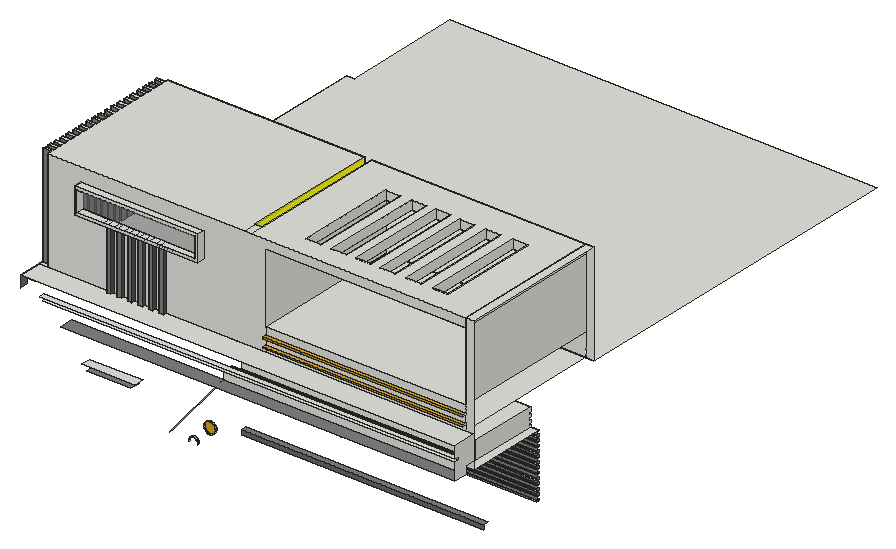
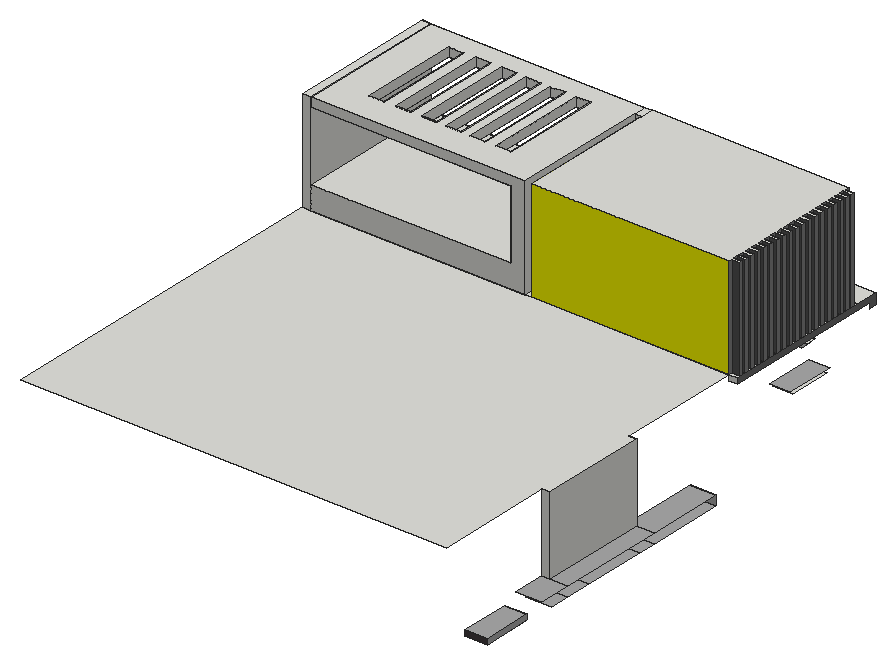
# SketchUp Ruby script. Lengths in inches.
U = 1.inch
M = Sketchup.active_model
def pt(a) = Geom::Point3d.new(a.map { |v| v * U })
def face(e, loops, mat)
  f = e.add_face(loops[0].map { |a| pt(a) })
  loops[1..].each { |l| e.add_face(l.map { |a| pt(a) }).erase! }
  f.material = f.back_material = mat if mat
  f
end
# faces: each face lists its corners as indices into pts; further lists are holes
def faces(e, pts, list, mat = nil) = list.each { |f| face(e, (f[0].is_a?(Array) ? f : [f]).map { |l| l.map { |i| pts[i] } }, mat) }
# xy, xz, yz: faces in a plane at the given z, y or x. An outline is a flat list of corners, or four numbers for a rectangle; further outlines are holes
def ring(l) = l.size == 4 ? [[l[0], l[1]], [l[2], l[1]], [l[2], l[3]], [l[0], l[3]]] : l.each_slice(2).to_a
def flat(e, list, mat, &to3) = list.each { |f| face(e, (f[0].is_a?(Array) ? f : [f]).map { |l| ring(l).map { |u, v| to3.(u, v) } }, mat) }
def xy(e, z, list, mat = nil) = flat(e, list, mat) { |x, y| [x, y, z] }
def xz(e, y, list, mat = nil) = flat(e, list, mat) { |x, z| [x, y, z] }
def yz(e, x, list, mat = nil) = flat(e, list, mat) { |y, z| [x, y, z] }
def lines(e, pts, list) = list.each { |a, b| e.add_line(pt(pts[a]), pt(pts[b])) }
# prism: a flat outline (further loops are holes) pulled along v
def prism(e, loops, v, mat = nil)
  f = face(e, loops, mat); d = Geom::Vector3d.new(v.map { |x| x * U })
  f.pushpull(f.normal.samedirection?(d) ? d.length : -d.length)
end
def box(e, o, s, mat = nil) = prism(e, [[o, [o[0] + s[0], o[1], o[2]], [o[0] + s[0], o[1] + s[1], o[2]], [o[0], o[1] + s[1], o[2]]]], [0, 0, s[2]], mat)
def at(x, y, z, deg = 0) = Geom::Transformation.translation(pt([x, y, z])) * Geom::Transformation.rotation(ORIGIN, Z_AXIS, deg.degrees)
def axes(o, x, y, z) = Geom::Transformation.new([*x, 0, *y, 0, *z, 0, *pt(o).to_a, 1])
def part(name) = M.definitions.add(name)
# library, detail: a bought-in or finely detailed component or shape, given as its bounding box
def library(name, o, s) = part(name).tap { |d| box(d.entities, o, s) }
def detail(e, o, s) = box(e.add_group.entities, o, s)
def put(e, d, t, mat = nil) = e.add_instance(d, t).tap { |i| i.material = mat if mat }
def group(e, t, mat = nil) = e.add_group.tap { |g| g.transformation = t; g.material = mat if mat }.entities
root = M.entities
M.materials.add("[0045_Goldenrod]").color = [218, 165, 32]
M.materials.add("[0056_Yellow]").color = [255, 255, 0]
M.materials.add("[0132_LightGray]").color = [169, 169, 169]
M.materials.add("[0133_Gray]").color = [128, 128, 128]
M.materials.add("[0134_DimGray]").color = [105, 105, 105]
M.materials.add("[0135_DarkGray]").color = [81, 81, 81]
M.materials.add("[Asphalt New]").color = [67, 60, 62]
M.materials.add("[Translucent Glass Gold]").color = [255, 254, 26]
M.materials["[Translucent Glass Gold]"].alpha = 0.6
M.materials.add("[Translucent Glass Gray]").color = [128, 128, 128]
M.materials["[Translucent Glass Gray]"].alpha = 0.5
xy(root,121,[[362.29,137.46,366.5,138.52]])
xy(root,121,[[271.01,137.46,362.29,138.52]],"[0133_Gray]")
xy(root,122.32,[[271.01,137.46,362.29,138.52],[362.29,137.46,366.5,138.52]])
xy(root,123.5,[[362.29,137.46,366.5,138.52]])
xy(root,123.5,[[271.01,137.46,362.29,138.52]],"[0133_Gray]")
xy(root,124.57,[[134.1875,319.63,140.3125,322.32],[134.1875,322.32,145.875,342.57],[134.1875,342.57,140.3125,345.26]],"[0132_LightGray]")
xy(root,124.82,[[271.01,137.46,362.29,138.52],[362.29,137.46,366.5,138.52]])
xy(root,125.14,[[143.25,239.14,145.875,245.77],[143.25,284.1,145.875,295.35]])
xy(root,125.14,[[132.5625,199.28,145.875,239.14],[132.5625,239.14,132.5625,248.5,145.875,248.5,145.875,245.77,143.25,245.77,143.25,239.14],[132.5625,248.5,145.875,281.37],[132.5625,281.37,132.5625,295.35,143.25,295.35,143.25,284.1,145.875,284.1,145.875,281.37],[132.5625,295.35,145.875,305.66]],"[0132_LightGray]")
xy(root,125.6875,[[241.18,103.28,366.5,105.72]],"[0133_Gray]")
xy(root,126,[[271.01,137.46,362.29,138.52],[362.29,137.46,366.5,138.52]])
xy(root,127.26,[[134.1875,319.63,145.875,345.26]],"[0132_LightGray]")
xy(root,127.32,[[271.01,137.46,362.29,138.52],[362.29,137.46,366.5,138.52]])
xy(root,128.5,[[271.01,137.46,362.29,138.52],[362.29,137.46,366.5,138.52]])
xy(root,129.82,[[271.01,137.46,362.29,138.52],[362.29,137.46,366.5,138.52]])
xy(root,130.21,[[132.5625,199.28,145.875,239.14],[132.5625,239.14,141.625,295.35],[132.5625,295.35,145.875,312.35]],"[0132_LightGray]")
xy(root,130.21,[[141.625,239.14,145.875,295.35]],"[Asphalt New]")
xy(root,131,[[271.01,137.46,362.29,138.52],[362.29,137.46,366.5,138.52]])
xy(root,132.32,[[271.01,137.46,362.29,138.52],[362.29,137.46,366.5,138.52]])
xy(root,133.5,[[271.01,137.46,362.29,138.52],[362.29,137.46,366.5,138.52]])
xy(root,134.82,[[271.01,137.46,362.29,138.52],[362.29,137.46,366.5,138.52]])
xy(root,136,[[271.01,137.46,362.29,138.52],[362.29,137.46,366.5,138.52]])
xy(root,136.72,[[174.32,86.4,197.1,91.46]],"[0133_Gray]")
xy(root,137.32,[[271.01,137.46,362.29,138.52],[362.29,137.46,366.5,138.52]])
xy(root,138.5,[[271.01,137.46,362.29,138.52],[362.29,137.46,366.5,138.52]])
xy(root,139.05,[[171.99,86.4,199.43,91.46]])
xy(root,139.82,[[271.01,137.46,362.29,138.52],[362.29,137.46,366.5,138.52]])
xy(root,141,[[271.01,137.46,362.29,138.52],[362.29,137.46,366.5,138.52]])
xy(root,142.32,[[271.01,137.46,362.29,138.52],[362.29,137.46,366.5,138.52]])
xy(root,143.5,[[271.01,137.46,362.29,138.52],[362.29,137.46,366.5,138.52]])
xy(root,144.82,[[241.18,129.9,271.01,137.46],[271.01,137.46,366.5,138.52]])
xy(root,146,[[241.18,137.46,362.29,138.52],[362.29,137.46,366.5,138.52]])
xy(root,147.32,[[241.18,137.46,366.5,138.52]])
xy(root,148.5,[[241.18,137.46,362.29,138.52],[362.29,137.46,366.5,138.52]])
xy(root,149.82,[[241.18,137.46,366.5,138.52]])
xy(root,151,[[241.18,137.46,362.29,138.52],[362.29,137.46,366.5,138.52]])
xy(root,152.32,[[241.18,137.46,366.5,138.52]])
xy(root,152.9375,[[135.375,124.36,145.875,146.21]])
xy(root,153.5,[[241.18,137.46,362.29,138.52],[362.29,137.46,366.5,138.52]])
xy(root,154.0625,[[241.18,96.65,241.18,103.2,362.29,103.2,362.29,138.52,366.5,138.52,366.5,96.65]])
xy(root,154.0625,[[162.7,84.4,366.5,91.46]],"[0133_Gray]")
xy(root,154.77,[[135.375,122.53,145.875,148.03]],"[0132_LightGray]")
xy(root,154.82,[[241.18,137.46,362.29,138.52]])
xy(root,156,[[241.18,137.46,362.29,138.52]])
xy(root,157.32,[[241.18,137.46,362.29,138.52]])
xy(root,158,[[241.18,91.46,366.5,96.65]])
xy(root,158.5,[[241.18,137.46,362.29,138.52]])
xy(root,159.82,[[241.18,137.46,362.29,138.52]])
xy(root,161.04,[[241.18,137.46,362.29,138.52]])
xy(root,162.8125,[[153.22,84.4,366.5,87.02]])
xy(root,163.35,[[241.18,103.2,362.29,138.52]])
xy(root,164.22,[[151.875,84.4,366.5,87.02]])
xy(root,167.52,[[141.625,88.32,145.875,174.26]])
xy(root,170.5625,[[141.625,84.4,366.5,84.4,366.5,96.65,207.27,96.65,207.27,95.08,204.95,95.08,204.95,96.65,201.83,96.65,201.83,95.08,199.52,95.08,199.52,96.65,196.39,96.65,196.39,95.08,194.08,95.08,194.08,96.65,190.96,96.65,190.96,95.08,188.64,95.08,188.64,96.65,185.52,96.65,185.52,95.08,183.2,95.08,183.2,96.65,180.08,96.65,180.08,95.08,177.77,95.08,177.77,96.65,141.625,96.65],[177.77,95.08,180.08,95.08,180.08,96.65,183.2,96.65,183.2,95.08,185.52,95.08,185.52,96.65,188.64,96.65,188.64,95.08,190.96,95.08,190.96,96.65,194.08,96.65,194.08,95.08,196.39,95.08,196.39,96.65,199.52,96.65,199.52,95.08,201.83,95.08,201.83,96.65,204.95,96.65,204.95,95.08,207.27,95.08,207.27,96.65,247.84,96.65,247.84,174.26,145.875,174.26,145.875,172.76,141.625,172.76,141.625,171.1875,145.875,171.1875,145.875,169.32,141.625,169.32,141.625,167.75,145.875,167.75,145.875,165.41,141.625,165.41,141.625,163.625,145.875,163.625,145.875,161.28,141.625,161.28,141.625,159.5,145.875,159.5,145.875,157.16,141.625,157.16,141.625,155.375,145.875,155.375,145.875,153.03,141.625,153.03,141.625,151.25,145.875,151.25,145.875,148.91,141.625,148.91,141.625,147.125,145.875,147.125,145.875,144.78,141.625,144.78,141.625,143,145.875,143,145.875,140.66,141.625,140.66,141.625,138.875,145.875,138.875,145.875,136.53,141.625,136.53,141.625,134.75,145.875,134.75,145.875,132.41,141.625,132.41,141.625,130.625,145.875,130.625,145.875,128.28,141.625,128.28,141.625,126.5,145.875,126.5,145.875,124.16,141.625,124.16,141.625,122.375,145.875,122.375,145.875,120.03,141.625,120.03,141.625,118.25,145.875,118.25,145.875,115.91,141.625,115.91,141.625,114.125,145.875,114.125,145.875,111.78,141.625,111.78,141.625,110,145.875,110,145.875,107.66,141.625,107.66,141.625,105.875,145.875,105.875,145.875,104.28,141.625,104.28,141.625,102.43,145.875,102.43,145.875,100.59,141.625,100.59,141.625,98.99,145.875,98.99,145.875,96.65,177.77,96.65],[141.625,96.65,145.875,98.99],[247.84,96.65,362.28,96.65,362.28,174.26,251.44,174.26,251.44,103.57,247.84,103.57],[141.625,100.59,145.875,102.43],
  [247.84,103.57,251.44,174.26],[141.625,104.28,145.875,105.875],[141.625,107.66,145.875,110],[141.625,111.78,145.875,114.125],[141.625,115.91,145.875,118.25],
  [141.625,120.03,145.875,122.375],[141.625,124.16,145.875,126.5],[141.625,128.28,145.875,130.625],[141.625,132.41,145.875,134.75],[141.625,136.53,145.875,138.875],
  [141.625,140.66,145.875,143],[141.625,144.78,145.875,147.125],[141.625,148.91,145.875,151.25],[141.625,153.03,145.875,155.375],[141.625,157.16,145.875,159.5],
  [141.625,161.28,145.875,163.625],[141.625,165.41,145.875,167.75],[141.625,169.32,145.875,171.1875],[141.625,172.76,145.875,174.26],[145.875,174.26,366.5,174.26,366.5,356.98,145.875,356.98,145.875,295.35,141.625,295.35,141.625,239.14,145.875,239.14]])
xy(root,173.38,[[258.73,94.58,362.28,96.65]],"[0045_Goldenrod]")
xy(root,174.23,[[258.73,94.58,362.28,96.65]],"[0045_Goldenrod]")
xy(root,177.9,[[258.73,94.58,362.28,96.65]],"[0045_Goldenrod]")
xy(root,178.83,[[258.73,94.58,362.28,96.65]],"[0045_Goldenrod]")
xy(root,182.48,[[258.73,96.65,362.28,174.26]])
xy(root,202.43,[[162.99,92.83,177.77,96.65],[177.77,92.83,180.08,95.08],[180.08,92.83,183.2,96.65],[183.2,92.83,185.52,95.08],[185.52,92.83,188.64,96.65],
  [188.64,92.83,190.96,95.08],[190.96,92.83,194.08,96.65],[194.08,92.83,196.39,95.08],[196.39,92.83,199.52,96.65],[199.52,92.83,201.83,95.08],
  [201.83,92.83,204.95,96.65],[204.95,92.83,207.27,95.08],[207.27,92.83,226.7,96.65]])
xy(root,203.71,[[164.27,92.83,177.77,96.65],[177.77,92.83,180.08,96.65],[180.08,92.83,183.2,96.65],[183.2,92.83,185.52,96.65],[185.52,92.83,188.64,96.65],
  [188.64,92.83,190.96,96.65],[190.96,92.83,194.08,96.65],[194.08,92.83,196.39,96.65],[196.39,92.83,199.52,96.65],[199.52,92.83,201.83,96.65],
  [201.83,92.83,204.95,96.65],[204.95,92.83,207.27,96.65],[207.27,92.83,225.43,96.65]])
xy(root,214.48,[[164.27,92.83,225.43,96.65]])
xy(root,215.75,[[162.99,92.83,226.7,96.65]])
xy(root,218.43,[[[258.73,96.65,362.3,174.26],[271.2,107.02,279.01,158.84],[284.45,107.02,292.26,158.84],[296.88,107.02,304.7,158.84],[309.7,107.02,317.51,158.84],[323.07,107.02,330.88,158.84],[336.82,107.02,344.63,158.84]]])
xy(root,223.125,[[145.875,96.65,247.84,96.65,247.84,174.26,145.875,174.26,145.875,172.76,141.625,172.76,141.625,171.1875,145.875,171.1875,145.875,169.32,141.625,169.32,141.625,167.75,145.875,167.75,145.875,165.41,141.625,165.41,141.625,163.625,145.875,163.625,145.875,161.28,141.625,161.28,141.625,159.5,145.875,159.5,145.875,157.16,141.625,157.16,141.625,155.375,145.875,155.375,145.875,153.03,141.625,153.03,141.625,151.25,145.875,151.25,145.875,148.91,141.625,148.91,141.625,147.125,145.875,147.125,145.875,144.78,141.625,144.78,141.625,143,145.875,143,145.875,140.66,141.625,140.66,141.625,138.875,145.875,138.875,145.875,136.53,141.625,136.53,141.625,134.75,145.875,134.75,145.875,132.41,141.625,132.41,141.625,130.625,145.875,130.625,145.875,128.28,141.625,128.28,141.625,126.5,145.875,126.5,145.875,124.16,141.625,124.16,141.625,122.375,145.875,122.375,145.875,120.03,141.625,120.03,141.625,118.25,145.875,118.25,145.875,115.91,141.625,115.91,141.625,114.125,145.875,114.125,145.875,111.78,141.625,111.78,141.625,110,145.875,110,145.875,107.66,141.625,107.66,141.625,105.875,145.875,105.875,145.875,104.28,141.625,104.28,141.625,102.43,145.875,102.43,145.875,100.59,141.625,100.59,141.625,98.99,145.875,98.99],[247.84,96.65,251.44,103.57],[[251.44,96.65,362.28,174.26],[271.2,107.02,279.01,158.84],[284.45,107.02,292.26,158.84],[296.88,107.02,304.7,158.84],[309.7,107.02,317.51,158.84],[323.07,107.02,330.88,158.84],[336.82,107.02,344.63,158.84]],[362.28,96.65,362.3,174.26],[362.3,96.65,366.5,174.26]])
xz(root,90.02,[[235.69,127.61,236.46,127.71,237.19,128.01,237.81,128.49,238.28,129.11,238.58,129.83,238.69,130.61,238.58,131.38,238.28,132.11,237.81,132.73,237.19,133.21,236.46,133.5,235.69,133.61,234.91,133.5,234.19,133.21,233.5625,132.73,233.09,132.11,232.79,131.38,232.69,130.61,232.79,129.83,233.09,129.11,233.5625,128.49,234.19,128.01,234.91,127.71]],"[0045_Goldenrod]")
xz(root,91.46,[[241.18,154.0625,366.5,158]])
xz(root,92.83,[[[162.99,202.43,226.7,215.75],[164.27,203.71,225.43,214.48]]])
xz(root,94.58,[[258.73,173.38,362.28,174.23],[258.73,177.9,362.28,178.83]],"[0045_Goldenrod]")
xz(root,95.08,[[177.77,170.5625,180.08,202.43],[183.2,170.5625,185.52,202.43],[188.64,170.5625,190.96,202.43],[194.08,170.5625,196.39,202.43],[199.52,170.5625,201.83,202.43],
  [204.95,170.5625,207.27,202.43]],"[0133_Gray]")
xz(root,96.65,[[241.18,154.0625,366.5,158],[145.875,170.5625,177.77,170.5625,177.77,202.43,162.99,202.43,162.99,215.75,226.7,215.75,226.7,202.43,207.27,202.43,207.27,170.5625,258.73,170.5625,258.73,218.43,362.28,218.43,362.28,223.125,145.875,223.125],[180.08,170.5625,183.2,202.43],[185.52,170.5625,188.64,202.43],[190.96,170.5625,194.08,202.43],
  [196.39,170.5625,199.52,202.43],[201.83,170.5625,204.95,202.43],[258.73,170.5625,362.28,173.38],[362.28,170.5625,366.5,170.5625,366.5,223.125,362.3,223.125,362.3,218.43,362.28,218.43],[258.73,174.23,362.28,177.9],
  [258.73,178.83,362.28,182.48],[362.28,218.43,362.3,223.125]])
xz(root,96.65,[[164.27,203.71,225.43,214.48]],"[Translucent Glass Gray]")
xz(root,98.99,[[141.625,170.5625,145.875,223.125]],"[0133_Gray]")
xz(root,100.59,[[141.625,170.5625,145.875,223.125]],"[0135_DarkGray]")
xz(root,102.43,[[141.625,170.5625,145.875,223.125]],"[0133_Gray]")
xz(root,103.2,[[241.18,154.0625,362.29,163.35]])
xz(root,103.28,[[241.18,123.39,366.5,125.6875]],"[0134_DimGray]")
xz(root,103.57,[[247.84,170.5625,251.44,223.125]])
xz(root,104.28,[[141.625,170.5625,145.875,223.125]],"[0135_DarkGray]")
xz(root,105.875,[[141.625,170.5625,145.875,223.125]],"[0133_Gray]")
xz(root,107.02,[[271.2,218.43,279.01,223.125],[284.45,218.43,292.26,223.125],[296.88,218.43,304.7,223.125],[309.7,218.43,317.51,223.125],[323.07,218.43,330.88,223.125],
  [336.82,218.43,344.63,223.125]])
xz(root,107.66,[[141.625,170.5625,145.875,223.125]],"[0135_DarkGray]")
xz(root,110,[[141.625,170.5625,145.875,223.125]],"[0133_Gray]")
xz(root,111.78,[[141.625,170.5625,145.875,223.125]],"[0135_DarkGray]")
xz(root,114.125,[[141.625,170.5625,145.875,223.125]],"[0133_Gray]")
xz(root,115.91,[[141.625,170.5625,145.875,223.125]],"[0135_DarkGray]")
xz(root,118.25,[[141.625,170.5625,145.875,223.125]],"[0133_Gray]")
xz(root,120.03,[[141.625,170.5625,145.875,223.125]],"[0135_DarkGray]")
xz(root,122.375,[[141.625,170.5625,145.875,223.125]],"[0133_Gray]")
xz(root,124.16,[[141.625,170.5625,145.875,223.125]],"[0135_DarkGray]")
xz(root,126.5,[[141.625,170.5625,145.875,223.125]],"[0133_Gray]")
xz(root,128.28,[[141.625,170.5625,145.875,223.125]],"[0135_DarkGray]")
xz(root,129.9,[[241.18,139.03,264.37,139.03,271.01,144.82,241.18,144.82]],"[0132_LightGray]")
xz(root,130.625,[[141.625,170.5625,145.875,223.125]],"[0133_Gray]")
xz(root,132.41,[[141.625,170.5625,145.875,223.125]],"[0135_DarkGray]")
xz(root,134.75,[[141.625,170.5625,145.875,223.125]],"[0133_Gray]")
xz(root,136.53,[[141.625,170.5625,145.875,223.125]],"[0135_DarkGray]")
xz(root,137.46,[[271.01,122.32,366.5,123.5],[271.01,124.82,366.5,126],[271.01,127.32,366.5,128.5],[271.01,129.82,366.5,131],[271.01,132.32,366.5,133.5],
  [271.01,134.82,366.5,136],[271.01,137.32,366.5,138.5],[271.01,139.82,366.5,141],[271.01,142.32,366.5,143.5],[241.18,144.82,366.5,146],
  [241.18,147.32,366.5,148.5],[241.18,149.82,366.5,151],[241.18,152.32,366.5,153.5],[241.18,154.82,362.29,156],[241.18,157.32,362.29,158.5],
  [241.18,159.82,362.29,161.04]],"[0133_Gray]")
xz(root,138.52,[[241.18,161.04,362.29,163.35]])
xz(root,138.52,[[271.01,121,366.5,122.32],[271.01,123.5,366.5,124.82],[271.01,126,366.5,127.32],[271.01,128.5,366.5,129.82],[271.01,131,366.5,132.32],
  [271.01,133.5,366.5,134.82],[271.01,136,366.5,137.32],[271.01,138.5,366.5,139.82],[271.01,141,366.5,142.32],[271.01,143.5,366.5,144.82],
  [241.18,146,366.5,147.32],[241.18,148.5,366.5,149.82],[241.18,151,366.5,152.32],[241.18,153.5,366.5,153.5,366.5,154.0625,362.29,154.0625,362.29,154.82,241.18,154.82],[241.18,156,362.29,157.32],
  [241.18,158.5,362.29,159.82]],"[0133_Gray]")
xz(root,138.875,[[141.625,170.5625,145.875,223.125]],"[0133_Gray]")
xz(root,140.66,[[141.625,170.5625,145.875,223.125]],"[0135_DarkGray]")
xz(root,143,[[141.625,170.5625,145.875,223.125]],"[0133_Gray]")
xz(root,144.78,[[141.625,170.5625,145.875,223.125]],"[0135_DarkGray]")
xz(root,147.125,[[141.625,170.5625,145.875,223.125]],"[0133_Gray]")
xz(root,148.91,[[141.625,170.5625,145.875,223.125]],"[0135_DarkGray]")
xz(root,151.25,[[141.625,170.5625,145.875,223.125]],"[0133_Gray]")
xz(root,153.03,[[141.625,170.5625,145.875,223.125]],"[0135_DarkGray]")
xz(root,155.375,[[141.625,170.5625,145.875,223.125]],"[0133_Gray]")
xz(root,157.16,[[141.625,170.5625,145.875,223.125]],"[0135_DarkGray]")
xz(root,158.84,[[271.2,218.43,279.01,223.125],[284.45,218.43,292.26,223.125],[296.88,218.43,304.7,223.125],[309.7,218.43,317.51,223.125],[323.07,218.43,330.88,223.125],
  [336.82,218.43,344.63,223.125]])
xz(root,159.5,[[141.625,170.5625,145.875,223.125]],"[0133_Gray]")
xz(root,161.28,[[141.625,170.5625,145.875,223.125]],"[0135_DarkGray]")
xz(root,163.625,[[141.625,170.5625,145.875,223.125]],"[0133_Gray]")
xz(root,165.41,[[141.625,170.5625,145.875,223.125]],"[0135_DarkGray]")
xz(root,167.75,[[141.625,170.5625,145.875,223.125]],"[0133_Gray]")
xz(root,169.32,[[141.625,170.5625,145.875,223.125]],"[0135_DarkGray]")
xz(root,171.1875,[[141.625,170.5625,145.875,223.125]],"[0133_Gray]")
xz(root,172.76,[[141.625,170.5625,145.875,223.125]],"[0135_DarkGray]")
xz(root,174.26,[[141.625,167.52,145.875,170.5625],[251.44,170.5625,251.44,223.125,362.28,223.125,362.28,218.43,258.73,218.43,258.73,182.48,362.28,182.48,362.28,170.5625],[362.28,170.5625,362.28,218.43,362.3,218.43,362.3,223.125,366.5,223.125,366.5,170.5625],[362.28,218.43,362.3,223.125]])
xz(root,174.26,[[145.875,170.5625,247.84,223.125]],"[0056_Yellow]")
xz(root,199.28,[[132.5625,125.14,145.875,130.21]],"[0132_LightGray]")
xz(root,239.14,[[141.625,130.21,145.875,170.5625]])
xz(root,295.35,[[141.625,130.21,145.875,170.5625]])
xz(root,319.63,[[134.1875,124.57,145.875,127.26]],"[0132_LightGray]")
xz(root,345.26,[[134.1875,124.57,145.875,127.26]],"[Asphalt New]")
yz(root,134.1875,[[319.63,124.57,345.26,127.26]],"[0132_LightGray]")
yz(root,141.625,[[239.14,130.21,295.35,170.5625]])
yz(root,141.625,[[98.99,170.5625,100.59,223.125],[102.43,170.5625,104.28,223.125],[105.875,170.5625,107.66,223.125],[110,170.5625,111.78,223.125],[114.125,170.5625,115.91,223.125],
  [118.25,170.5625,120.03,223.125],[122.375,170.5625,124.16,223.125],[126.5,170.5625,128.28,223.125],[130.625,170.5625,132.41,223.125],[134.75,170.5625,136.53,223.125],
  [138.875,170.5625,140.66,223.125],[143,170.5625,144.78,223.125],[147.125,170.5625,148.91,223.125],[151.25,170.5625,153.03,223.125],[155.375,170.5625,157.16,223.125],
  [159.5,170.5625,161.28,223.125],[163.625,170.5625,165.41,223.125],[167.75,170.5625,169.32,223.125],[171.1875,170.5625,172.76,223.125]],"[0133_Gray]")
yz(root,141.625,[[84.4,164.64,84.4,170.5625,174.26,170.5625,174.26,167.52,88.32,167.52,88.32,164.64]],"[0134_DimGray]")
yz(root,145.875,[[201.67,125.14,229.97,127.58],[245.77,125.14,284.1,127.87]])
yz(root,145.875,[[96.65,170.5625,98.99,223.125],[100.59,170.5625,102.43,223.125],[104.28,170.5625,105.875,223.125],[107.66,170.5625,110,223.125],[111.78,170.5625,114.125,223.125],
  [115.91,170.5625,118.25,223.125],[120.03,170.5625,122.375,223.125],[124.16,170.5625,126.5,223.125],[128.28,170.5625,130.625,223.125],[132.41,170.5625,134.75,223.125],
  [136.53,170.5625,138.875,223.125],[140.66,170.5625,143,223.125],[144.78,170.5625,147.125,223.125],[148.91,170.5625,151.25,223.125],[153.03,170.5625,155.375,223.125],
  [157.16,170.5625,159.5,223.125],[161.28,170.5625,163.625,223.125],[165.41,170.5625,167.75,223.125],[169.32,170.5625,171.1875,223.125],[172.76,170.5625,174.26,223.125]],"[0133_Gray]")
yz(root,162.99,[[92.83,202.43,96.65,215.75]])
yz(root,164.27,[[92.83,203.71,96.65,214.48]])
yz(root,177.77,[[95.08,170.5625,96.65,202.43]],"[0133_Gray]")
yz(root,180.08,[[95.08,170.5625,96.65,202.43]],"[0135_DarkGray]")
yz(root,183.2,[[95.08,170.5625,96.65,202.43]],"[0133_Gray]")
yz(root,185.52,[[95.08,170.5625,96.65,202.43]],"[0135_DarkGray]")
yz(root,188.64,[[95.08,170.5625,96.65,202.43]],"[0133_Gray]")
yz(root,190.96,[[95.08,170.5625,96.65,202.43]],"[0135_DarkGray]")
yz(root,194.08,[[95.08,170.5625,96.65,202.43]],"[0133_Gray]")
yz(root,196.39,[[95.08,170.5625,96.65,202.43]],"[0135_DarkGray]")
yz(root,199.52,[[95.08,170.5625,96.65,202.43]],"[0133_Gray]")
yz(root,201.83,[[95.08,170.5625,96.65,202.43]],"[0135_DarkGray]")
yz(root,204.95,[[95.08,170.5625,96.65,202.43]],"[0133_Gray]")
yz(root,207.27,[[95.08,170.5625,96.65,202.43]],"[0135_DarkGray]")
yz(root,225.43,[[92.83,203.71,96.65,214.48]])
yz(root,226.7,[[92.83,202.43,96.65,215.75]])
yz(root,247.84,[[103.57,170.5625,174.26,223.125]],"[Translucent Glass Gold]")
yz(root,251.44,[[103.57,170.5625,174.26,223.125]])
yz(root,258.73,[[94.58,173.38,96.65,174.23],[94.58,177.9,96.65,178.83],[96.65,182.48,174.26,218.43]])
yz(root,271.01,[[129.83,121,138.52,122.32],[129.83,122.32,137.46,123.5],[129.83,123.5,138.52,124.82],[129.83,124.82,137.46,126],[129.83,126,138.52,127.32],
  [129.83,127.32,137.46,128.5],[129.83,128.5,138.52,129.82],[129.83,129.82,137.46,131],[129.83,131,138.52,132.32],[129.83,132.32,137.46,133.5],
  [129.83,133.5,138.52,134.82],[129.83,134.82,137.46,136],[129.83,136,138.52,137.32],[129.83,137.32,137.46,138.5],[129.83,138.5,138.52,139.82],
  [129.83,139.82,137.46,141],[129.83,141,138.52,142.32],[129.83,142.32,137.46,143.5],[129.83,143.5,138.52,144.82]])
yz(root,271.2,[[107.02,218.43,158.84,223.125]])
yz(root,279.01,[[107.02,218.43,158.84,223.125]])
yz(root,284.45,[[107.02,218.43,158.84,223.125]])
yz(root,292.26,[[107.02,218.43,158.84,223.125]])
yz(root,296.88,[[107.02,218.43,158.84,223.125]])
yz(root,304.7,[[107.02,218.43,158.84,223.125]])
yz(root,309.7,[[107.02,218.43,158.84,223.125]])
yz(root,317.51,[[107.02,218.43,158.84,223.125]])
yz(root,323.07,[[107.02,218.43,158.84,223.125]])
yz(root,330.88,[[107.02,218.43,158.84,223.125]])
yz(root,336.82,[[107.02,218.43,158.84,223.125]])
yz(root,344.63,[[107.02,218.43,158.84,223.125]])
yz(root,362.28,[[94.58,173.38,96.65,174.23],[94.58,177.9,96.65,178.83],[96.65,182.48,174.26,223.125]])
yz(root,362.29,[[103.2,154.0625,103.2,163.35,138.52,163.35,138.52,161.04,137.46,161.04,137.46,159.82,138.52,159.82,138.52,158.5,137.46,158.5,137.46,157.32,138.52,157.32,138.52,156,137.46,156,137.46,154.82,138.52,154.82,138.52,154.0625]])
yz(root,362.3,[[96.65,218.43,174.26,223.125]])
yz(root,366.5,[[84.4,154.0625,91.46,154.0625,91.46,158,96.65,158,96.65,170.5625,84.4,170.5625,84.4,164.22,87.02,164.22,87.02,162.8125,84.4,162.8125]])
p = [[224.88,89.33,121.23],[224.96,89.33,120.65],[224.96,90.15,120.65],[224.88,90.15,121.23],[229.31,89.33,120.65],[229.38,89.33,121.23],
  [229.38,90.15,121.23],[229.31,90.15,120.65],[224.96,89.33,121.8125],[224.96,90.15,121.8125],[229.31,89.33,121.8125],[229.31,90.15,121.8125],
  [241.18,91.46,154.0625],[214.91,91.46,121.45],[214.91,89.33,121.45],[241.18,89.33,154.0625],[225.19,89.33,122.36],[225.19,90.15,122.36],
  [229.08,89.33,122.36],[229.08,90.15,122.36],[225.54,89.33,122.82],[225.54,90.15,122.82],[228.72,89.33,122.82],[228.72,90.15,122.82],
  [226.01,89.33,123.18],[226.01,90.15,123.18],[228.26,89.33,123.18],[228.26,90.15,123.18],[226.55,89.33,123.4],[226.55,90.15,123.4],
  [227.72,89.33,123.4],[227.72,90.15,123.4],[227.13,89.33,123.48],[227.13,90.15,123.48],[234.91,89.33,127.71],[235.69,89.33,127.61],
  [235.69,90.02,127.61],[234.91,90.02,127.71],[236.46,89.33,127.71],[236.46,90.02,127.71],[234.19,89.33,128.01],[234.19,90.02,128.01],
  [237.19,89.33,128.01],[237.19,90.02,128.01],[233.5625,89.33,128.49],[233.5625,90.02,128.49],[237.81,89.33,128.49],[237.81,90.02,128.49],
  [233.09,89.33,129.11],[233.09,90.02,129.11],[238.28,89.33,129.11],[238.28,90.02,129.11],[232.79,89.33,129.83],[232.79,90.02,129.83],
  [238.58,89.33,129.83],[238.58,90.02,129.83],[232.69,89.33,130.61],[232.69,90.02,130.61],[238.69,89.33,130.61],[238.69,90.02,130.61],
  [232.79,89.33,131.38],[232.79,90.02,131.38],[238.58,89.33,131.38],[238.58,90.02,131.38],[233.09,89.33,132.11],[233.09,90.02,132.11],
  [238.28,89.33,132.11],[238.28,90.02,132.11],[233.5625,89.33,132.73],[233.5625,90.02,132.73],[237.81,89.33,132.73],[237.81,90.02,132.73],
  [234.19,89.33,133.21],[234.19,90.02,133.21],[237.19,89.33,133.21],[237.19,90.02,133.21],[234.91,89.33,133.5],[234.91,90.02,133.5],
  [236.46,89.33,133.5],[236.46,90.02,133.5],[235.69,89.33,133.61],[235.69,90.02,133.61],[264.37,129.83,139.03],[271.01,129.83,144.82],
  [271.01,129.9,144.82],[264.37,129.9,139.03]]
faces(root,p,[[0,1,2,3],[4,5,6,7],[8,0,3,9],[5,10,11,6],[12,13,14,15],[16,8,9,17],[10,18,19,11],[20,16,17,21],
  [18,22,23,19],[24,20,21,25],[22,26,27,23],[28,24,25,29],[26,30,31,27],[32,28,29,33],[30,32,33,31],[34,35,36,37],
  [35,38,39,36],[40,34,37,41],[38,42,43,39],[44,40,41,45],[42,46,47,43],[48,44,45,49],[46,50,51,47],[52,48,49,53],
  [50,54,55,51],[56,52,53,57],[54,58,59,55],[60,56,57,61],[58,62,63,59],[64,60,61,65],[62,66,67,63],[68,64,65,69],
  [66,70,71,67],[72,68,69,73],[70,74,75,71],[76,72,73,77],[74,78,79,75],[80,76,77,81],[78,80,81,79],[82,83,84,85]])
